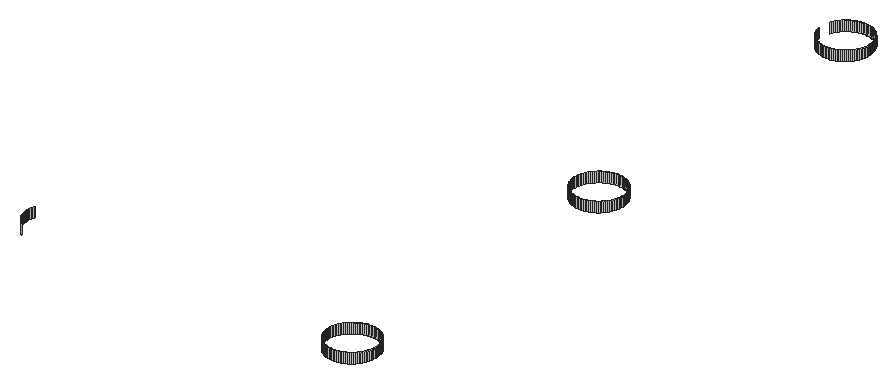
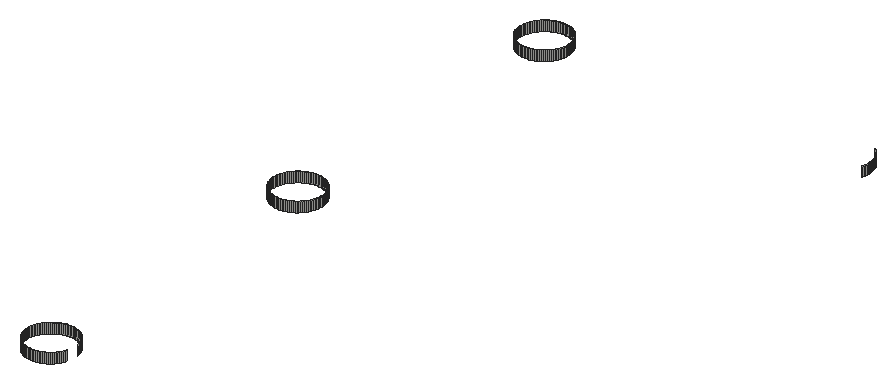
# SketchUp Ruby script. Lengths in inches.
U = 1.inch
M = Sketchup.active_model
def pt(a) = Geom::Point3d.new(a.map { |v| v * U })
def face(e, loops, mat)
  f = e.add_face(loops[0].map { |a| pt(a) })
  loops[1..].each { |l| e.add_face(l.map { |a| pt(a) }).erase! }
  f.material = f.back_material = mat if mat
  f
end
# faces: each face lists its corners as indices into pts; further lists are holes
def faces(e, pts, list, mat = nil) = list.each { |f| face(e, (f[0].is_a?(Array) ? f : [f]).map { |l| l.map { |i| pts[i] } }, mat) }
# xy, xz, yz: faces in a plane at the given z, y or x. An outline is a flat list of corners, or four numbers for a rectangle; further outlines are holes
def ring(l) = l.size == 4 ? [[l[0], l[1]], [l[2], l[1]], [l[2], l[3]], [l[0], l[3]]] : l.each_slice(2).to_a
def flat(e, list, mat, &to3) = list.each { |f| face(e, (f[0].is_a?(Array) ? f : [f]).map { |l| ring(l).map { |u, v| to3.(u, v) } }, mat) }
def xy(e, z, list, mat = nil) = flat(e, list, mat) { |x, y| [x, y, z] }
def xz(e, y, list, mat = nil) = flat(e, list, mat) { |x, z| [x, y, z] }
def yz(e, x, list, mat = nil) = flat(e, list, mat) { |y, z| [x, y, z] }
def lines(e, pts, list) = list.each { |a, b| e.add_line(pt(pts[a]), pt(pts[b])) }
# prism: a flat outline (further loops are holes) pulled along v
def prism(e, loops, v, mat = nil)
  f = face(e, loops, mat); d = Geom::Vector3d.new(v.map { |x| x * U })
  f.pushpull(f.normal.samedirection?(d) ? d.length : -d.length)
end
def box(e, o, s, mat = nil) = prism(e, [[o, [o[0] + s[0], o[1], o[2]], [o[0] + s[0], o[1] + s[1], o[2]], [o[0], o[1] + s[1], o[2]]]], [0, 0, s[2]], mat)
def at(x, y, z, deg = 0) = Geom::Transformation.translation(pt([x, y, z])) * Geom::Transformation.rotation(ORIGIN, Z_AXIS, deg.degrees)
def axes(o, x, y, z) = Geom::Transformation.new([*x, 0, *y, 0, *z, 0, *pt(o).to_a, 1])
def part(name) = M.definitions.add(name)
# library, detail: a bought-in or finely detailed component or shape, given as its bounding box
def library(name, o, s) = part(name).tap { |d| box(d.entities, o, s) }
def detail(e, o, s) = box(e.add_group.entities, o, s)
def put(e, d, t, mat = nil) = e.add_instance(d, t).tap { |i| i.material = mat if mat }
def group(e, t, mat = nil) = e.add_group.tap { |g| g.transformation = t; g.material = mat if mat }.entities
root = M.entities
xz(root,34,[[370.5625,231.53,370.9375,234]])
xz(root,46,[[370.5625,231.53,370.9375,234]])
xz(root,111,[[370.5625,231.53,370.9375,234]])
xz(root,123,[[370.5625,231.53,370.9375,234]])
xz(root,188,[[370.5625,231.53,370.9375,234]])
xz(root,200,[[370.5625,231.53,370.9375,234]])
yz(root,289.5625,[[39.8125,231.53,40.1875,234]])
yz(root,364.75,[[39.8125,231.53,40.1875,234],[116.8125,231.53,117.1875,234]])
yz(root,376.75,[[39.8125,231.53,40.1875,234],[116.8125,231.53,117.1875,234],[193.8125,231.53,194.1875,234]])
p = [[370.19,34.03,231.53],[369.8125,34.07,231.53],[369.8125,34.07,234],[370.19,34.03,234],[370.5625,34,231.53],[370.5625,34,234],
  [371.31,34.03,231.53],[370.9375,34,231.53],[370.9375,34,234],[371.31,34.03,234],[371.6875,34.07,231.53],[371.6875,34.07,234],
  [369.44,34.14,231.53],[369.08,34.24,231.53],[369.08,34.24,234],[369.44,34.14,234],[372.06,34.14,231.53],[372.06,34.14,234],
  [372.42,34.24,231.53],[372.42,34.24,234],[368.72,34.35,231.53],[368.72,34.35,234],[372.78,34.35,231.53],[372.78,34.35,234],
  [368.37,34.49,231.53],[368.37,34.49,234],[373.13,34.49,231.53],[373.13,34.49,234],[368.03,34.65,231.53],[368.03,34.65,234],
  [373.47,34.65,231.53],[373.47,34.65,234],[367.7,34.84,231.53],[367.7,34.84,234],[373.8,34.84,231.53],[373.8,34.84,234],
  [367.38,35.04,231.53],[367.38,35.04,234],[374.12,35.04,231.53],[374.12,35.04,234],[292.1875,35.04,231.53],[291.88,35.26,231.53],
  [291.88,35.26,234],[292.1875,35.04,234],[367.07,35.26,231.53],[367.07,35.26,234],[374.43,35.26,231.53],[374.43,35.26,234],
  [291.59,35.5,231.53],[291.59,35.5,234],[366.78,35.5,231.53],[366.78,35.5,234],[374.72,35.5,231.53],[374.72,35.5,234],
  [291.32,35.76,231.53],[291.32,35.76,234],[366.51,35.76,231.53],[366.51,35.76,234],[374.99,35.76,231.53],[374.99,35.76,234],
  [291.06,36.03,231.53],[291.06,36.03,234],[366.25,36.03,231.53],[366.25,36.03,234],[375.25,36.03,231.53],[375.25,36.03,234],
  [290.82,36.32,231.53],[290.82,36.32,234],[366.01,36.32,231.53],[366.01,36.32,234],[375.49,36.32,231.53],[375.49,36.32,234],
  [290.6,36.63,231.53],[290.6,36.63,234],[365.79,36.63,231.53],[365.79,36.63,234],[375.71,36.63,231.53],[375.71,36.63,234],
  [290.4,36.95,231.53],[290.4,36.95,234],[365.59,36.95,231.53],[365.59,36.95,234],[375.91,36.95,231.53],[375.91,36.95,234],
  [290.21,37.28,231.53],[290.21,37.28,234],[365.4,37.28,231.53],[365.4,37.28,234],[376.1,37.28,231.53],[376.1,37.28,234],
  [290.05,37.62,231.53],[290.05,37.62,234],[365.24,37.62,231.53],[365.24,37.62,234],[376.26,37.62,231.53],[376.26,37.62,234],
  [289.92,37.97,231.53],[289.92,37.97,234],[365.1,37.97,231.53],[365.1,37.97,234],[376.4,37.97,231.53],[376.4,37.97,234],
  [289.8,38.33,231.53],[289.8,38.33,234],[364.99,38.33,231.53],[364.99,38.33,234],[376.51,38.33,231.53],[376.51,38.33,234],
  [289.7,38.69,231.53],[289.7,38.69,234],[364.89,38.69,231.53],[364.89,38.69,234],[376.61,38.69,231.53],[376.61,38.69,234],
  [289.63,39.0625,231.53],[289.63,39.0625,234],[364.82,39.0625,231.53],[364.82,39.0625,234],[376.68,39.0625,231.53],[376.68,39.0625,234],
  [289.59,39.44,231.53],[289.59,39.44,234],[364.78,39.44,231.53],[364.78,39.44,234],[376.72,39.44,231.53],[376.72,39.44,234],
  [289.5625,39.8125,231.53],[289.5625,39.8125,234],[364.75,39.8125,231.53],[364.75,39.8125,234],[376.75,39.8125,231.53],[376.75,39.8125,234],
  [289.5625,40.1875,231.53],[289.59,40.56,231.53],[289.59,40.56,234],[289.5625,40.1875,234],[364.75,40.1875,231.53],[364.78,40.56,231.53],
  [364.78,40.56,234],[364.75,40.1875,234],[376.72,40.56,231.53],[376.75,40.1875,231.53],[376.75,40.1875,234],[376.72,40.56,234],
  [289.63,40.9375,231.53],[289.63,40.9375,234],[364.82,40.9375,231.53],[364.82,40.9375,234],[376.68,40.9375,231.53],[376.68,40.9375,234],
  [289.7,41.31,231.53],[289.7,41.31,234],[364.89,41.31,231.53],[364.89,41.31,234],[376.61,41.31,231.53],[376.61,41.31,234],
  [289.8,41.67,231.53],[289.8,41.67,234],[364.99,41.67,231.53],[364.99,41.67,234],[376.51,41.67,231.53],[376.51,41.67,234],
  [289.92,42.03,231.53],[289.92,42.03,234],[365.1,42.03,231.53],[365.1,42.03,234],[376.4,42.03,231.53],[376.4,42.03,234],
  [365.24,42.38,231.53],[365.24,42.38,234],[376.26,42.38,231.53],[376.26,42.38,234],[365.4,42.72,231.53],[365.4,42.72,234],
  [376.1,42.72,231.53],[376.1,42.72,234],[365.59,43.05,231.53],[365.59,43.05,234],[375.91,43.05,231.53],[375.91,43.05,234],
  [365.79,43.37,231.53],[365.79,43.37,234],[375.71,43.37,231.53],[375.71,43.37,234],[366.01,43.68,231.53],[366.01,43.68,234],
  [375.49,43.68,231.53],[375.49,43.68,234],[366.25,43.97,231.53],[366.25,43.97,234],[375.25,43.97,231.53],[375.25,43.97,234],
  [366.51,44.24,231.53],[366.51,44.24,234],[374.99,44.24,231.53],[374.99,44.24,234],[366.78,44.5,231.53],[366.78,44.5,234],
  [374.72,44.5,231.53],[374.72,44.5,234],[367.07,44.74,231.53],[367.07,44.74,234],[374.43,44.74,231.53],[374.43,44.74,234],
  [367.38,44.96,231.53],[367.38,44.96,234],[374.12,44.96,231.53],[374.12,44.96,234],[367.7,45.16,231.53],[367.7,45.16,234],
  [373.8,45.16,231.53],[373.8,45.16,234],[368.03,45.35,231.53],[368.03,45.35,234],[373.47,45.35,231.53],[373.47,45.35,234],
  [368.37,45.51,231.53],[368.37,45.51,234],[373.13,45.51,231.53],[373.13,45.51,234],[368.72,45.65,231.53],[368.72,45.65,234],
  [372.78,45.65,231.53],[372.78,45.65,234],[369.08,45.76,231.53],[369.08,45.76,234],[372.42,45.76,231.53],[372.42,45.76,234],
  [369.44,45.86,231.53],[369.44,45.86,234],[372.06,45.86,231.53],[372.06,45.86,234],[369.8125,45.93,231.53],[369.8125,45.93,234],
  [370.19,45.97,231.53],[370.19,45.97,234],[371.31,45.97,231.53],[371.6875,45.93,231.53],[371.6875,45.93,234],[371.31,45.97,234],
  [370.5625,46,231.53],[370.5625,46,234],[370.9375,46,231.53],[370.9375,46,234],[370.19,111.03,231.53],[369.8125,111.07,231.53],
  [369.8125,111.07,234],[370.19,111.03,234],[370.5625,111,231.53],[370.5625,111,234],[371.31,111.03,231.53],[370.9375,111,231.53],
  [370.9375,111,234],[371.31,111.03,234],[371.6875,111.07,231.53],[371.6875,111.07,234],[369.44,111.14,231.53],[369.08,111.24,231.53],
  [369.08,111.24,234],[369.44,111.14,234],[372.06,111.14,231.53],[372.06,111.14,234],[372.42,111.24,231.53],[372.42,111.24,234],
  [368.72,111.35,231.53],[368.72,111.35,234],[372.78,111.35,231.53],[372.78,111.35,234],[368.37,111.49,231.53],[368.37,111.49,234],
  [373.13,111.49,231.53],[373.13,111.49,234],[368.03,111.65,231.53],[368.03,111.65,234],[373.47,111.65,231.53],[373.47,111.65,234],
  [367.7,111.84,231.53],[367.7,111.84,234],[373.8,111.84,231.53],[373.8,111.84,234],[367.38,112.04,231.53],[367.38,112.04,234],
  [374.12,112.04,231.53],[374.12,112.04,234],[367.07,112.26,231.53],[367.07,112.26,234],[374.43,112.26,231.53],[374.43,112.26,234],
  [366.78,112.5,231.53],[366.78,112.5,234],[374.72,112.5,231.53],[374.72,112.5,234],[366.51,112.76,231.53],[366.51,112.76,234],
  [374.99,112.76,231.53],[374.99,112.76,234],[366.25,113.03,231.53],[366.25,113.03,234],[375.25,113.03,231.53],[375.25,113.03,234],
  [366.01,113.32,231.53],[366.01,113.32,234],[375.49,113.32,231.53],[375.49,113.32,234],[365.79,113.63,231.53],[365.79,113.63,234],
  [375.71,113.63,231.53],[375.71,113.63,234],[365.59,113.95,231.53],[365.59,113.95,234],[375.91,113.95,231.53],[375.91,113.95,234],
  [365.4,114.28,231.53],[365.4,114.28,234],[376.1,114.28,231.53],[376.1,114.28,234],[365.24,114.62,231.53],[365.24,114.62,234],
  [376.26,114.62,231.53],[376.26,114.62,234],[365.1,114.97,231.53],[365.1,114.97,234],[376.4,114.97,231.53],[376.4,114.97,234],
  [364.99,115.33,231.53],[364.99,115.33,234],[376.51,115.33,231.53],[376.51,115.33,234],[364.89,115.69,231.53],[364.89,115.69,234],
  [376.61,115.69,231.53],[376.61,115.69,234],[364.82,116.0625,231.53],[364.82,116.0625,234],[376.68,116.0625,231.53],[376.68,116.0625,234],
  [364.78,116.44,231.53],[364.78,116.44,234],[376.72,116.44,231.53],[376.72,116.44,234],[364.75,116.8125,231.53],[364.75,116.8125,234],
  [376.75,116.8125,231.53],[376.75,116.8125,234],[364.75,117.1875,231.53],[364.78,117.56,231.53],[364.78,117.56,234],[364.75,117.1875,234],
  [376.72,117.56,231.53],[376.75,117.1875,231.53],[376.75,117.1875,234],[376.72,117.56,234],[364.82,117.9375,231.53],[364.82,117.9375,234],
  [376.68,117.9375,231.53],[376.68,117.9375,234],[364.89,118.31,231.53],[364.89,118.31,234],[376.61,118.31,231.53],[376.61,118.31,234],
  [364.99,118.67,231.53],[364.99,118.67,234],[376.51,118.67,231.53],[376.51,118.67,234],[365.1,119.03,231.53],[365.1,119.03,234],
  [376.4,119.03,231.53],[376.4,119.03,234],[365.24,119.38,231.53],[365.24,119.38,234],[376.26,119.38,231.53],[376.26,119.38,234],
  [365.4,119.72,231.53],[365.4,119.72,234],[376.1,119.72,231.53],[376.1,119.72,234],[365.59,120.05,231.53],[365.59,120.05,234],
  [375.91,120.05,231.53],[375.91,120.05,234],[365.79,120.37,231.53],[365.79,120.37,234],[375.71,120.37,231.53],[375.71,120.37,234],
  [366.01,120.68,231.53],[366.01,120.68,234],[375.49,120.68,231.53],[375.49,120.68,234],[366.25,120.97,231.53],[366.25,120.97,234],
  [375.25,120.97,231.53],[375.25,120.97,234],[366.51,121.24,231.53],[366.51,121.24,234],[374.99,121.24,231.53],[374.99,121.24,234],
  [366.78,121.5,231.53],[366.78,121.5,234],[374.72,121.5,231.53],[374.72,121.5,234],[367.07,121.74,231.53],[367.07,121.74,234],
  [374.43,121.74,231.53],[374.43,121.74,234],[367.38,121.96,231.53],[367.38,121.96,234],[374.12,121.96,231.53],[374.12,121.96,234],
  [367.7,122.16,231.53],[367.7,122.16,234],[373.8,122.16,231.53],[373.8,122.16,234],[368.03,122.35,231.53],[368.03,122.35,234],
  [373.47,122.35,231.53],[373.47,122.35,234],[368.37,122.51,231.53],[368.37,122.51,234],[373.13,122.51,231.53],[373.13,122.51,234],
  [368.72,122.65,231.53],[368.72,122.65,234],[372.78,122.65,231.53],[372.78,122.65,234],[369.08,122.76,231.53],[369.08,122.76,234],
  [372.42,122.76,231.53],[372.42,122.76,234],[369.44,122.86,231.53],[369.44,122.86,234],[372.06,122.86,231.53],[372.06,122.86,234],
  [369.8125,122.93,231.53],[369.8125,122.93,234],[370.19,122.97,231.53],[370.19,122.97,234],[371.31,122.97,231.53],[371.6875,122.93,231.53],
  [371.6875,122.93,234],[371.31,122.97,234],[370.5625,123,231.53],[370.5625,123,234],[370.9375,123,231.53],[370.9375,123,234],
  [370.19,188.03,231.53],[369.8125,188.07,231.53],[369.8125,188.07,234],[370.19,188.03,234],[370.5625,188,231.53],[370.5625,188,234],
  [371.31,188.03,231.53],[370.9375,188,231.53],[370.9375,188,234],[371.31,188.03,234],[371.6875,188.07,231.53],[371.6875,188.07,234],
  [369.44,188.14,231.53],[369.08,188.24,231.53],[369.08,188.24,234],[369.44,188.14,234],[372.06,188.14,231.53],[372.06,188.14,234],
  [372.42,188.24,231.53],[372.42,188.24,234],[368.72,188.35,231.53],[368.72,188.35,234],[372.78,188.35,231.53],[372.78,188.35,234],
  [368.37,188.49,231.53],[368.37,188.49,234],[373.13,188.49,231.53],[373.13,188.49,234],[368.03,188.65,231.53],[368.03,188.65,234],
  [373.47,188.65,231.53],[373.47,188.65,234],[367.7,188.84,231.53],[367.7,188.84,234],[373.8,188.84,231.53],[373.8,188.84,234],
  [367.38,189.04,231.53],[367.38,189.04,234],[374.12,189.04,231.53],[374.12,189.04,234],[367.07,189.26,231.53],[367.07,189.26,234],
  [374.43,189.26,231.53],[374.43,189.26,234],[366.78,189.5,231.53],[366.78,189.5,234],[374.72,189.5,231.53],[374.72,189.5,234],
  [366.51,189.76,231.53],[366.51,189.76,234],[374.99,189.76,231.53],[374.99,189.76,234],[366.25,190.03,231.53],[366.25,190.03,234],
  [375.25,190.03,231.53],[375.25,190.03,234],[366.01,190.32,231.53],[366.01,190.32,234],[375.49,190.32,231.53],[375.49,190.32,234],
  [365.79,190.63,231.53],[365.79,190.63,234],[375.71,190.63,231.53],[375.71,190.63,234],[365.59,190.95,231.53],[365.59,190.95,234],
  [375.91,190.95,231.53],[375.91,190.95,234],[365.4,191.28,231.53],[365.4,191.28,234],[376.1,191.28,231.53],[376.1,191.28,234],
  [365.24,191.62,231.53],[365.24,191.62,234],[376.26,191.62,231.53],[376.26,191.62,234],[365.1,191.97,231.53],[365.1,191.97,234],
  [376.4,191.97,231.53],[376.4,191.97,234],[364.99,192.33,231.53],[364.99,192.33,234],[376.51,192.33,231.53],[376.51,192.33,234],
  [364.89,192.69,231.53],[364.89,192.69,234],[376.61,192.69,231.53],[376.61,192.69,234],[364.82,193.0625,231.53],[364.82,193.0625,234],
  [376.68,193.0625,231.53],[376.68,193.0625,234],[376.72,193.44,231.53],[376.72,193.44,234],[376.75,193.8125,231.53],[376.75,193.8125,234],
  [376.72,194.56,231.53],[376.75,194.1875,231.53],[376.75,194.1875,234],[376.72,194.56,234],[376.68,194.9375,231.53],[376.68,194.9375,234],
  [376.61,195.31,231.53],[376.61,195.31,234],[376.51,195.67,231.53],[376.51,195.67,234],[376.4,196.03,231.53],[376.4,196.03,234],
  [365.1,196.03,231.53],[365.24,196.38,231.53],[365.24,196.38,234],[365.1,196.03,234],[376.26,196.38,231.53],[376.26,196.38,234],
  [365.4,196.72,231.53],[365.4,196.72,234],[376.1,196.72,231.53],[376.1,196.72,234],[365.59,197.05,231.53],[365.59,197.05,234],
  [375.91,197.05,231.53],[375.91,197.05,234],[365.79,197.37,231.53],[365.79,197.37,234],[375.71,197.37,231.53],[375.71,197.37,234],
  [366.01,197.68,231.53],[366.01,197.68,234],[375.49,197.68,231.53],[375.49,197.68,234],[366.25,197.97,231.53],[366.25,197.97,234],
  [375.25,197.97,231.53],[375.25,197.97,234],[366.51,198.24,231.53],[366.51,198.24,234],[374.99,198.24,231.53],[374.99,198.24,234],
  [366.78,198.5,231.53],[366.78,198.5,234],[374.72,198.5,231.53],[374.72,198.5,234],[367.07,198.74,231.53],[367.07,198.74,234],
  [374.43,198.74,231.53],[374.43,198.74,234],[367.38,198.96,231.53],[367.38,198.96,234],[374.12,198.96,231.53],[374.12,198.96,234],
  [367.7,199.16,231.53],[367.7,199.16,234],[373.8,199.16,231.53],[373.8,199.16,234],[368.03,199.35,231.53],[368.03,199.35,234],
  [373.47,199.35,231.53],[373.47,199.35,234],[368.37,199.51,231.53],[368.37,199.51,234],[373.13,199.51,231.53],[373.13,199.51,234],
  [368.72,199.65,231.53],[368.72,199.65,234],[372.78,199.65,231.53],[372.78,199.65,234],[369.08,199.76,231.53],[369.08,199.76,234],
  [372.42,199.76,231.53],[372.42,199.76,234],[369.44,199.86,231.53],[369.44,199.86,234],[372.06,199.86,231.53],[372.06,199.86,234],
  [369.8125,199.93,231.53],[369.8125,199.93,234],[370.19,199.97,231.53],[370.19,199.97,234],[371.31,199.97,231.53],[371.6875,199.93,231.53],
  [371.6875,199.93,234],[371.31,199.97,234],[370.5625,200,231.53],[370.5625,200,234],[370.9375,200,231.53],[370.9375,200,234]]
faces(root,p,[[0,1,2,3],[4,0,3,5],[6,7,8,9],[10,6,9,11],[12,13,14,15],[1,12,15,2],[16,10,11,17],[18,16,17,19],
  [13,20,21,14],[22,18,19,23],[20,24,25,21],[26,22,23,27],[24,28,29,25],[30,26,27,31],[28,32,33,29],[34,30,31,35],
  [32,36,37,33],[38,34,35,39],[40,41,42,43],[36,44,45,37],[46,38,39,47],[41,48,49,42],[44,50,51,45],[52,46,47,53],
  [48,54,55,49],[50,56,57,51],[58,52,53,59],[54,60,61,55],[56,62,63,57],[64,58,59,65],[60,66,67,61],[62,68,69,63],
  [70,64,65,71],[66,72,73,67],[68,74,75,69],[76,70,71,77],[72,78,79,73],[74,80,81,75],[82,76,77,83],[78,84,85,79],
  [80,86,87,81],[88,82,83,89],[84,90,91,85],[86,92,93,87],[94,88,89,95],[90,96,97,91],[92,98,99,93],[100,94,95,101],
  [96,102,103,97],[98,104,105,99],[106,100,101,107],[102,108,109,103],[104,110,111,105],[112,106,107,113],[108,114,115,109],[110,116,117,111],
  [118,112,113,119],[114,120,121,115],[116,122,123,117],[124,118,119,125],[120,126,127,121],[122,128,129,123],[130,124,125,131],[132,133,134,135],
  [136,137,138,139],[140,141,142,143],[133,144,145,134],[137,146,147,138],[148,140,143,149],[144,150,151,145],[146,152,153,147],[154,148,149,155],
  [150,156,157,151],[152,158,159,153],[160,154,155,161],[156,162,163,157],[158,164,165,159],[166,160,161,167],[164,168,169,165],[170,166,167,171],
  [168,172,173,169],[174,170,171,175],[172,176,177,173],[178,174,175,179],[176,180,181,177],[182,178,179,183],[180,184,185,181],[186,182,183,187],
  [184,188,189,185],[190,186,187,191],[188,192,193,189],[194,190,191,195],[192,196,197,193],[198,194,195,199],[196,200,201,197],[202,198,199,203],
  [200,204,205,201],[206,202,203,207],[204,208,209,205],[210,206,207,211],[208,212,213,209],[214,210,211,215],[212,216,217,213],[218,214,215,219],
  [216,220,221,217],[222,218,219,223],[220,224,225,221],[226,222,223,227],[224,228,229,225],[230,226,227,231],[228,232,233,229],[232,234,235,233],
  [236,237,238,239],[237,230,231,238],[234,240,241,235],[242,236,239,243],[244,245,246,247],[248,244,247,249],[250,251,252,253],[254,250,253,255],
  [256,257,258,259],[245,256,259,246],[260,254,255,261],[262,260,261,263],[257,264,265,258],[266,262,263,267],[264,268,269,265],[270,266,267,271],
  [268,272,273,269],[274,270,271,275],[272,276,277,273],[278,274,275,279],[276,280,281,277],[282,278,279,283],[280,284,285,281],[286,282,283,287],
  [284,288,289,285],[290,286,287,291],[288,292,293,289],[294,290,291,295],[292,296,297,293],[298,294,295,299],[296,300,301,297],[302,298,299,303],
  [300,304,305,301],[306,302,303,307],[304,308,309,305],[310,306,307,311],[308,312,313,309],[314,310,311,315],[312,316,317,313],[318,314,315,319],
  [316,320,321,317],[322,318,319,323],[320,324,325,321],[326,322,323,327],[324,328,329,325],[330,326,327,331],[328,332,333,329],[334,330,331,335],
  [332,336,337,333],[338,334,335,339],[336,340,341,337],[342,338,339,343],[344,345,346,347],[348,349,350,351],[345,352,353,346],[354,348,351,355],
  [352,356,357,353],[358,354,355,359],[356,360,361,357],[362,358,359,363],[360,364,365,361],[366,362,363,367],[364,368,369,365],[370,366,367,371],
  [368,372,373,369],[374,370,371,375],[372,376,377,373],[378,374,375,379],[376,380,381,377],[382,378,379,383],[380,384,385,381],[386,382,383,387],
  [384,388,389,385],[390,386,387,391],[388,392,393,389],[394,390,391,395],[392,396,397,393],[398,394,395,399],[396,400,401,397],[402,398,399,403],
  [400,404,405,401],[406,402,403,407],[404,408,409,405],[410,406,407,411],[408,412,413,409],[414,410,411,415],[412,416,417,413],[418,414,415,419],
  [416,420,421,417],[422,418,419,423],[420,424,425,421],[426,422,423,427],[424,428,429,425],[430,426,427,431],[428,432,433,429],[432,434,435,433],
  [436,437,438,439],[437,430,431,438],[434,440,441,435],[442,436,439,443],[444,445,446,447],[448,444,447,449],[450,451,452,453],[454,450,453,455],
  [456,457,458,459],[445,456,459,446],[460,454,455,461],[462,460,461,463],[457,464,465,458],[466,462,463,467],[464,468,469,465],[470,466,467,471],
  [468,472,473,469],[474,470,471,475],[472,476,477,473],[478,474,475,479],[476,480,481,477],[482,478,479,483],[480,484,485,481],[486,482,483,487],
  [484,488,489,485],[490,486,487,491],[488,492,493,489],[494,490,491,495],[492,496,497,493],[498,494,495,499],[496,500,501,497],[502,498,499,503],
  [500,504,505,501],[506,502,503,507],[504,508,509,505],[510,506,507,511],[508,512,513,509],[514,510,511,515],[512,516,517,513],[518,514,515,519],
  [516,520,521,517],[522,518,519,523],[520,524,525,521],[526,522,523,527],[524,528,529,525],[530,526,527,531],[528,532,533,529],[534,530,531,535],
  [536,534,535,537],[538,536,537,539],[540,541,542,543],[544,540,543,545],[546,544,545,547],[548,546,547,549],[550,548,549,551],[552,553,554,555],
  [556,550,551,557],[553,558,559,554],[560,556,557,561],[558,562,563,559],[564,560,561,565],[562,566,567,563],[568,564,565,569],[566,570,571,567],
  [572,568,569,573],[570,574,575,571],[576,572,573,577],[574,578,579,575],[580,576,577,581],[578,582,583,579],[584,580,581,585],[582,586,587,583],
  [588,584,585,589],[586,590,591,587],[592,588,589,593],[590,594,595,591],[596,592,593,597],[594,598,599,595],[600,596,597,601],[598,602,603,599],
  [604,600,601,605],[602,606,607,603],[608,604,605,609],[606,610,611,607],[612,608,609,613],[610,614,615,611],[616,612,613,617],[614,618,619,615],
  [618,620,621,619],[622,623,624,625],[623,616,617,624],[620,626,627,621],[628,622,625,629]])
